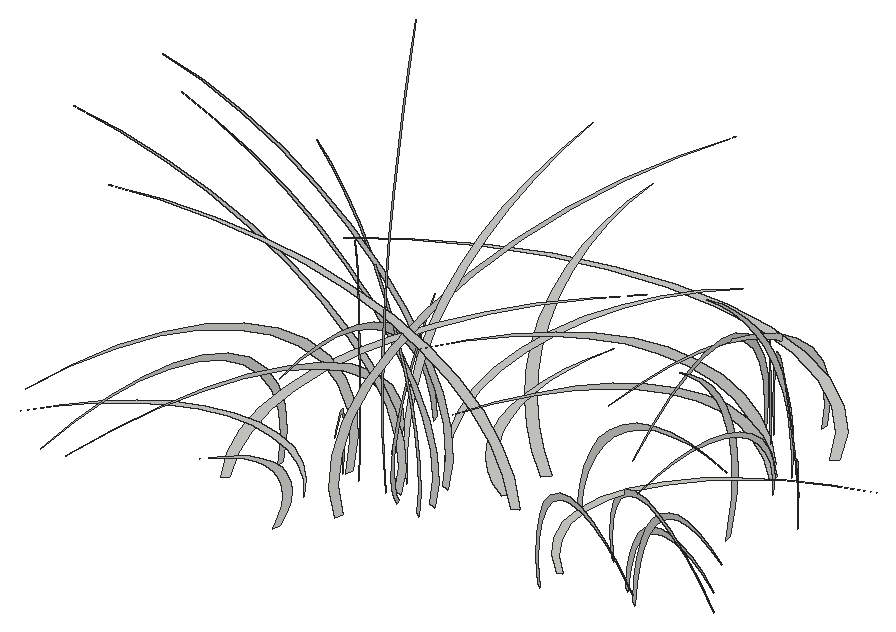
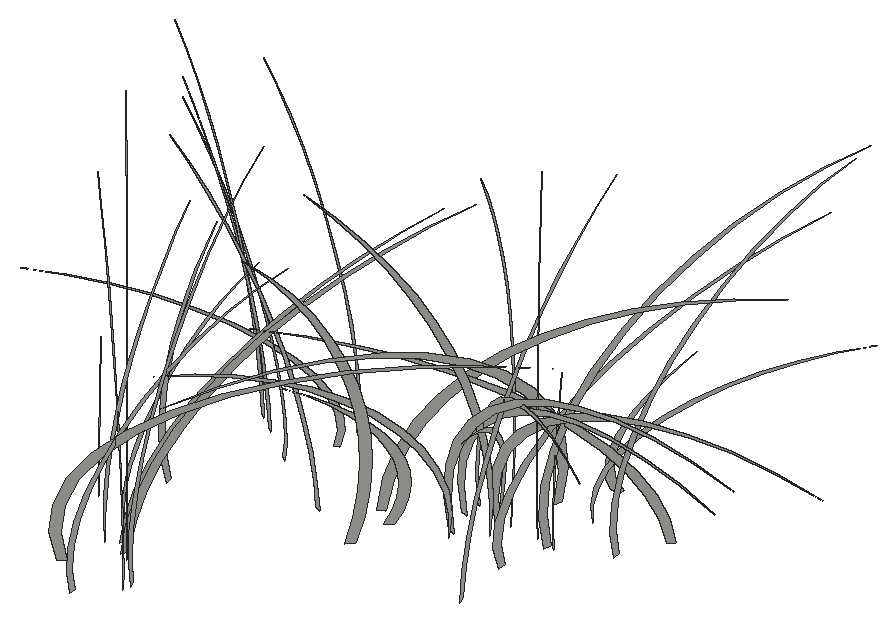
# SketchUp Ruby script. Lengths in inches.
U = 1.inch
M = Sketchup.active_model
def pt(a) = Geom::Point3d.new(a.map { |v| v * U })
def face(e, loops, mat)
  f = e.add_face(loops[0].map { |a| pt(a) })
  loops[1..].each { |l| e.add_face(l.map { |a| pt(a) }).erase! }
  f.material = f.back_material = mat if mat
  f
end
# faces: each face lists its corners as indices into pts; further lists are holes
def faces(e, pts, list, mat = nil) = list.each { |f| face(e, (f[0].is_a?(Array) ? f : [f]).map { |l| l.map { |i| pts[i] } }, mat) }
# xy, xz, yz: faces in a plane at the given z, y or x. An outline is a flat list of corners, or four numbers for a rectangle; further outlines are holes
def ring(l) = l.size == 4 ? [[l[0], l[1]], [l[2], l[1]], [l[2], l[3]], [l[0], l[3]]] : l.each_slice(2).to_a
def flat(e, list, mat, &to3) = list.each { |f| face(e, (f[0].is_a?(Array) ? f : [f]).map { |l| ring(l).map { |u, v| to3.(u, v) } }, mat) }
def xy(e, z, list, mat = nil) = flat(e, list, mat) { |x, y| [x, y, z] }
def xz(e, y, list, mat = nil) = flat(e, list, mat) { |x, z| [x, y, z] }
def yz(e, x, list, mat = nil) = flat(e, list, mat) { |y, z| [x, y, z] }
def lines(e, pts, list) = list.each { |a, b| e.add_line(pt(pts[a]), pt(pts[b])) }
# prism: a flat outline (further loops are holes) pulled along v
def prism(e, loops, v, mat = nil)
  f = face(e, loops, mat); d = Geom::Vector3d.new(v.map { |x| x * U })
  f.pushpull(f.normal.samedirection?(d) ? d.length : -d.length)
end
def box(e, o, s, mat = nil) = prism(e, [[o, [o[0] + s[0], o[1], o[2]], [o[0] + s[0], o[1] + s[1], o[2]], [o[0], o[1] + s[1], o[2]]]], [0, 0, s[2]], mat)
def at(x, y, z, deg = 0) = Geom::Transformation.translation(pt([x, y, z])) * Geom::Transformation.rotation(ORIGIN, Z_AXIS, deg.degrees)
def axes(o, x, y, z) = Geom::Transformation.new([*x, 0, *y, 0, *z, 0, *pt(o).to_a, 1])
def part(name) = M.definitions.add(name)
# library, detail: a bought-in or finely detailed component or shape, given as its bounding box
def library(name, o, s) = part(name).tap { |d| box(d.entities, o, s) }
def detail(e, o, s) = box(e.add_group.entities, o, s)
def put(e, d, t, mat = nil) = e.add_instance(d, t).tap { |i| i.material = mat if mat }
def group(e, t, mat = nil) = e.add_group.tap { |g| g.transformation = t; g.material = mat if mat }.entities
root = M.entities
g1 = group(root,at(58.66,562.84,0.02))
p = [[0.12,-0.92,0],[0.05,-0.41,0],[0,0,1.75],[0.02,-0.16,3.51],[0.11,-0.9,5.24],[0.27,-2.18,6.89],
  [0.5,-3.98,8.42],[0.79,-6.26,9.8],[1.13,-8.95,10.98],[1.51,-12,11.95],[1.93,-15.32,12.67],[2.37,-18.83,13.13],
  [2.83,-22.45,13.32],[3.28,-26.08,13.23],[2.84,-22.52,13.25],[2.39,-18.99,13],[1.96,-15.57,12.5],[1.56,-12.36,11.75],
  [1.19,-9.41,10.78],[0.86,-6.8,9.6],[0.58,-4.59,8.25],[0.36,-2.83,6.75],[0.2,-1.56,5.13],[0.1,-0.81,3.44],
  [0.07,-0.59,1.72]]
faces(g1,p,[[0,1,2,3,4,5,6,7,8,9,10,11,12,13,14,15,16,17,18,19,20,21,22,23,24]])
g2 = group(root,at(62.45,564.45,0.02))
p = [[-0.1,-0.92,0],[-0.05,-0.41,0],[0,0,2.0625],[-0.02,-0.17,4.13],[-0.1,-0.9,6.16],[-0.24,-2.1875,8.1],
  [-0.44,-3.99,9.91],[-0.69,-6.27,11.52],[-0.99,-8.97,12.92],[-1.33,-12.02,14.05],[-1.69,-15.34,14.9],[-2.08,-18.86,15.45],
  [-2.48,-22.49,15.67],[-2.88,-26.13,15.5625],[-2.49,-22.56,15.58],[-2.1,-19.02,15.29],[-1.72,-15.6,14.71],[-1.37,-12.38,13.83],
  [-1.04,-9.43,12.68],[-0.75,-6.81,11.3],[-0.51,-4.6,9.7],[-0.3125,-2.84,7.9375],[-0.17,-1.5625,6.04],[-0.09,-0.81,4.05],
  [-0.07,-0.59,2.02]]
faces(g2,p,[[0,1,2,3,4,5,6,7,8,9,10,11,12,13,14,15,16,17,18,19,20,21,22,23,24]])
g3 = group(root,at(62.45,564.45,0.02))
p = [[-0.1,-0.92,0],[-0.05,-0.41,0],[0,0,2.0625],[-0.02,-0.17,4.13],[-0.1,-0.9,6.16],[-0.24,-2.1875,8.1],
  [-0.44,-3.99,9.91],[-0.69,-6.27,11.52],[-0.99,-8.97,12.92],[-1.33,-12.02,14.05],[-1.69,-15.34,14.9],[-2.08,-18.86,15.45],
  [-2.48,-22.49,15.67],[-2.88,-26.13,15.5625],[-2.49,-22.56,15.58],[-2.1,-19.02,15.29],[-1.72,-15.6,14.71],[-1.37,-12.38,13.83],
  [-1.04,-9.43,12.68],[-0.75,-6.81,11.3],[-0.51,-4.6,9.7],[-0.3125,-2.84,7.9375],[-0.17,-1.5625,6.04],[-0.09,-0.81,4.05],
  [-0.07,-0.59,2.02]]
faces(g3,p,[[0,1,2,3,4,5,6,7,8,9,10,11,12,13,14,15,16,17,18,19,20,21,22,23,24]])
g4 = group(root,at(62.21,560.12,0.02))
p = [[-9.23,-14.04,8.41],[-7.99,-12.15,8.36],[-6.77,-10.29,8.15],[-5.59,-8.5,7.8],[-4.48,-6.8125,7.32],[-3.46,-5.26,6.7],
  [-2.54,-3.86,5.97],[-1.75,-2.66,5.13],[-1.09,-1.67,4.2],[-0.59,-0.9,3.21],[-0.25,-0.39,2.16],[-0.08,-0.125,1.09],
  [-0.08,-0.125,0],[0,0,1.11],[-0.11,-0.16,2.21],[-0.4,-0.61,3.29],[-0.88,-1.34,4.32],[-1.53,-2.33,5.28],
  [-2.33,-3.55,6.14],[-3.27,-4.98,6.88],[-4.33,-6.59,7.5],[-5.48,-8.34,7.97],[-6.7,-10.19,8.28],[-7.96,-12.11,8.43]]
faces(g4,p,[[0,1,2,3,4,5,6,7,8,9,10,11,12,13,14,15,16,17,18,19,20,21,22,23]])
g5 = group(root,at(78.25,560.67,0.02))
p = [[0.65,-0.5,0],[0.29,-0.22,0],[0,0,1.55],[0.12,-0.09,3.11],[0.63,-0.49,4.64],[1.54,-1.19,6.1],
  [2.81,-2.18,7.45],[4.41,-3.42,8.67],[6.31,-4.9,9.72],[8.45,-6.5625,10.57],[10.79,-8.38,11.21],[13.27,-10.3,11.62],
  [15.82,-12.28,11.79],[18.375,-14.26,11.71],[15.86,-12.31,11.72],[13.375,-10.38,11.5],[10.97,-8.52,11.0625],[8.71,-6.76,10.4],
  [6.63,-5.15,9.54],[4.79,-3.72,8.5],[3.24,-2.51,7.3],[1.99,-1.55,5.97],[1.1,-0.85,4.54],[0.57,-0.44,3.05],
  [0.42,-0.32,1.52]]
faces(g5,p,[[0,1,2,3,4,5,6,7,8,9,10,11,12,13,14,15,16,17,18,19,20,21,22,23,24]])
g6 = group(root,at(63,567.87,0.02))
p = [[-0.06,-0.99,0],[-0.03,-0.44,0],[0,0,1.49],[-0.01,-0.18,2.99],[-0.06,-0.97,4.45],[-0.14,-2.36,5.86],
  [-0.26,-4.3,7.16],[-0.4,-6.76,8.33],[-0.58,-9.67,9.33],[-0.77,-12.96,10.15],[-0.99,-16.54,10.77],[-1.22,-20.34,11.16],
  [-1.45,-24.24,11.32],[-1.68,-28.17,11.24],[-1.45,-24.32,11.26],[-1.23,-20.51,11.05],[-1.01,-16.82,10.625],[-0.8,-13.35,9.99],
  [-0.61,-10.16,9.16],[-0.4375,-7.35,8.16],[-0.3,-4.96,7.01],[-0.18,-3.06,5.73],[-0.1,-1.69,4.36],[-0.05,-0.87,2.93],
  [-0.04,-0.64,1.46]]
faces(g6,p,[[0,1,2,3,4,5,6,7,8,9,10,11,12,13,14,15,16,17,18,19,20,21,22,23,24]])
g7 = group(root,at(63.25,557.55,0.02))
p = [[-0.91,-7.12,6.7],[-0.75,-5.82,6.27],[-0.6,-4.64,5.81],[-0.46,-3.6,5.31],[-0.35,-2.71,4.77],[-0.25,-1.97,4.21],
  [-0.18,-1.39,3.63],[-0.125,-0.98,3.03],[-0.09,-0.74,2.43],[-0.09,-0.67,1.8125],[-0.1,-0.77,1.2],[-0.13,-1.05,0.59],
  [-0.19,-1.49,0],[-0.12,-0.92,0],[-0.05,-0.42,0.6],[-0.01,-0.11,1.22],[0,0,1.84],[-0.01,-0.08,2.47],
  [-0.04,-0.35,3.09],[-0.1,-0.81,3.69],[-0.1875,-1.45,4.28],[-0.29,-2.27,4.84],[-0.42,-3.26,5.37],[-0.57,-4.41,5.86],
  [-0.73,-5.7,6.3]]
faces(g7,p,[[0,1,2,3,4,5,6,7,8,9,10,11,12,13,14,15,16,17,18,19,20,21,22,23,24]])
g8 = group(root,at(84,562.16,0.02))
p = [[14.52,-11.27,13.58],[16.72,-12.98,13.9375],[14.59,-11.33,13.5],[12.54,-9.74,12.9],[10.59,-8.22,12.14],[8.75,-6.79,11.23],
  [7.05,-5.48,10.18],[5.51,-4.28,8.99],[4.14,-3.22,7.7],[2.97,-2.3,6.29],[1.99,-1.55,4.81],[1.23,-0.95,3.25],
  [0.69,-0.54,1.64],[0.38,-0.29,0],[0,0,0],[0.26,-0.2,1.68],[0.76,-0.59,3.33],[1.51,-1.17,4.92],
  [2.49,-1.93,6.45],[3.69,-2.87,7.875],[5.1,-3.96,9.19],[6.7,-5.2,10.38],[8.46,-6.57,11.43],[10.37,-8.05,12.3125],
  [12.4,-9.625,13.03]]
faces(g8,p,[[0,1,2,3,4,5,6,7,8,9,10,11,12,13,14,15,16,17,18,19,20,21,22,23,24]])
g9 = group(root,at(82.65,563.21,0.02))
p = [[14.52,-11.27,10.95],[16.72,-12.98,11.24],[14.59,-11.33,10.89],[12.54,-9.74,10.41],[10.59,-8.22,9.79],[8.75,-6.79,9.06],
  [7.05,-5.48,8.21],[5.51,-4.28,7.25],[4.14,-3.22,6.21],[2.97,-2.3,5.08],[1.99,-1.55,3.875],[1.23,-0.95,2.62],
  [0.69,-0.54,1.32],[0.38,-0.29,0],[0,0,0],[0.26,-0.2,1.36],[0.76,-0.59,2.69],[1.51,-1.17,3.97],
  [2.49,-1.93,5.2],[3.69,-2.87,6.35],[5.1,-3.96,7.41],[6.7,-5.2,8.37],[8.46,-6.57,9.21],[10.37,-8.05,9.93],
  [12.4,-9.625,10.51]]
faces(g9,p,[[0,1,2,3,4,5,6,7,8,9,10,11,12,13,14,15,16,17,18,19,20,21,22,23,24]])
g10 = group(root,at(79.64,565.54,0.02))
p = [[0.69,-0.54,0],[0.31,-0.24,0],[0,0,1.32],[0.125,-0.1,2.64],[0.68,-0.53,3.94],[1.65,-1.28,5.18],
  [3.01,-2.34,6.33],[4.74,-3.68,7.37],[6.77,-5.26,8.26],[9.07,-7.04,8.99],[11.59,-8.99,9.53],[14.24,-11.06,9.875],
  [16.98,-13.18,10.02],[19.73,-15.3125,9.95],[17.03,-13.22,9.96],[14.36,-11.15,9.78],[11.78,-9.14,9.4],[9.35,-7.26,8.84],
  [7.12,-5.53,8.11],[5.15,-3.99,7.22],[3.47,-2.7,6.2],[2.14,-1.66,5.07],[1.18,-0.92,3.86],[0.61,-0.47,2.59],
  [0.45,-0.35,1.29]]
faces(g10,p,[[0,1,2,3,4,5,6,7,8,9,10,11,12,13,14,15,16,17,18,19,20,21,22,23,24]])
g11 = group(root,at(62.26,571.81,0.02))
p = [[6.07,-19.87,14.56],[6.99,-22.87,14.94],[6.1,-19.96,14.48],[5.25,-17.16,13.83],[4.43,-14.49,13.02],[3.66,-11.97,12.04],
  [2.95,-9.65,10.91],[2.31,-7.54,9.64],[1.73,-5.67,8.25],[1.24,-4.06,6.75],[0.83,-2.72,5.15],[0.51,-1.68,3.49],
  [0.29,-0.94,1.76],[0.16,-0.52,0],[0,0,0],[0.11,-0.35,1.8],[0.32,-1.04,3.57],[0.63,-2.07,5.28],
  [1.04,-3.41,6.91],[1.55,-5.05,8.44],[2.13,-6.98,9.85],[2.8,-9.16,11.13],[3.54,-11.58,12.25],[4.34,-14.1875,13.2],
  [5.1875,-16.96,13.97]]
faces(g11,p,[[0,1,2,3,4,5,6,7,8,9,10,11,12,13,14,15,16,17,18,19,20,21,22,23,24]])
g12 = group(root,at(62.8125,564.18,0.02))
p = [[0.57,-0.76,0],[0.25,-0.34,1.67],[0.0625,-0.09,3.36],[0,0,5.0625],[0.0625,-0.08,6.76],[0.25,-0.33,8.45],
  [0.5625,-0.75,10.12],[1,-1.34,11.77],[1.56,-2.08,13.4],[2.23,-2.99,14.98],[3.03,-4.05,16.53],[3.93,-5.26,18.02],
  [4.95,-6.62,19.46],[3.99,-5.34,18],[3.14,-4.2,16.49],[2.39,-3.19,14.9375],[1.74,-2.33,13.35],[1.2,-1.61,11.73],
  [0.77,-1.03,10.08],[0.46,-0.61,8.42],[0.25,-0.34,6.74],[0.16,-0.21,5.05],[0.18,-0.24,3.36],[0.32,-0.43,1.68]]
faces(g12,p,[[0,1,2,3,4,5,6,7,8,9,10,11,12,13,14,15,16,17,18,19,20,21,22,23]])
g13 = group(root,at(61.19,564.82,0.02))
p = [[5.52,-7.72,6.7],[4.47,-6.25,6.27],[3.52,-4.92,5.81],[2.68,-3.75,5.31],[1.96,-2.74,4.77],[1.37,-1.91,4.21],
  [0.9,-1.26,3.63],[0.57,-0.79,3.03],[0.37,-0.52,2.43],[0.31,-0.44,1.8125],[0.4,-0.56,1.2],[0.62,-0.87,0.59],
  [0.98,-1.37,0],[0.74,-1.03,0],[0.33,-0.46,0.59],[0.07,-0.1,1.19],[-0.04,0.05,1.81],[0.01,-0.02,2.43],
  [0.21,-0.3,3.04],[0.5625,-0.79,3.65],[1.0625,-1.49,4.23],[1.7,-2.38,4.8],[2.48,-3.47,5.33],[3.38,-4.73,5.83],
  [4.4,-6.15,6.29]]
faces(g13,p,[[0,1,2,3,4,5,6,7,8,9,10,11,12,13,14,15,16,17,18,19,20,21,22,23,24]])
g14 = group(root,at(72.51,566.4,0.02))
p = [[-19.18,-7.98,16.73],[-22.08,-9.1875,17.17],[-19.27,-8.02,16.64],[-16.57,-6.9,15.9],[-13.98,-5.82,14.96],[-11.56,-4.8125,13.84],
  [-9.32,-3.88,12.54],[-7.28,-3.03,11.08],[-5.47,-2.28,9.48],[-3.92,-1.63,7.76],[-2.63,-1.09,5.92],[-1.625,-0.68,4.01],
  [-0.91,-0.38,2.02],[-0.5,-0.21,0],[0,0,0],[-0.34,-0.14,2.07],[-1.01,-0.42,4.1],[-1.99,-0.83,6.07],
  [-3.29,-1.37,7.94],[-4.88,-2.03,9.7],[-6.74,-2.81,11.33],[-8.85,-3.68,12.79],[-11.18,-4.65,14.08],[-13.7,-5.7,15.17],
  [-16.375,-6.82,16.0625]]
faces(g14,p,[[0,1,2,3,4,5,6,7,8,9,10,11,12,13,14,15,16,17,18,19,20,21,22,23,24]])
g15 = group(root,at(74.89,568.54,0.02))
p = [[16.23,-8.63,12.88],[18.68,-9.93,13.22],[16.3125,-8.67,12.8125],[14.02,-7.45,12.24],[11.84,-6.29,11.52],[9.78,-5.2,10.66],
  [7.88,-4.19,9.66],[6.16,-3.28,8.53],[4.63,-2.46,7.3],[3.32,-1.76,5.97],[2.23,-1.18,4.5625],[1.375,-0.73,3.08],
  [0.77,-0.41,1.56],[0.42,-0.22,0],[0,0,0],[0.29,-0.15,1.6],[0.85,-0.45,3.16],[1.6875,-0.9,4.67],
  [2.78,-1.48,6.12],[4.13,-2.2,7.47],[5.7,-3.03,8.72],[7.49,-3.98,9.85],[9.46,-5.03,10.84],[11.59,-6.16,11.68],
  [13.86,-7.37,12.37]]
faces(g15,p,[[0,1,2,3,4,5,6,7,8,9,10,11,12,13,14,15,16,17,18,19,20,21,22,23,24]])
g16 = group(root,at(78.28,562.01,0.02))
p = [[0.625,0.24,0],[0.28,0.11,0],[0,0,1.1],[0.11,0.04,2.21],[0.61,0.24,3.29],[1.49,0.57,4.33],
  [2.72,1.04,5.29],[4.28,1.64,6.15],[6.11,2.34,6.9],[8.19,3.14,7.51],[10.46,4.01,7.96],[12.86,4.93,8.25],
  [15.33,5.88,8.37],[17.8125,6.83,8.3125],[15.375,5.9,8.32],[12.97,4.97,8.17],[10.64,4.08,7.85],[8.4375,3.24,7.39],
  [6.43,2.46,6.77],[4.65,1.78,6.03],[3.14,1.2,5.18],[1.93,0.74,4.24],[1.07,0.41,3.23],[0.55,0.21,2.16],
  [0.4,0.16,1.08]]
faces(g16,p,[[0,1,2,3,4,5,6,7,8,9,10,11,12,13,14,15,16,17,18,19,20,21,22,23,24]])
g17 = group(root,at(57.05,558.92,0.02))
p = [[17.17,11.7,12.375],[19.76,13.47,12.7],[17.25,11.76,12.31],[14.83,10.11,11.76],[12.52,8.53,11.07],[10.35,7.05,10.23],
  [8.34,5.68,9.27],[6.52,4.44,8.2],[4.9,3.34,7.01],[3.51,2.39,5.74],[2.35,1.6,4.38],[1.45,0.99,2.96],
  [0.82,0.56,1.5],[0.45,0.3,0],[0,0,0],[0.3,0.21,1.53],[0.9,0.61,3.03],[1.78,1.22,4.49],
  [2.95,2.01,5.875],[4.37,2.98,7.18],[6.03,4.11,8.375],[7.92,5.4,9.46],[10,6.82,10.41],[12.26,8.36,11.22],
  [14.66,9.99,11.88]]
faces(g17,p,[[0,1,2,3,4,5,6,7,8,9,10,11,12,13,14,15,16,17,18,19,20,21,22,23,24]])
g18 = group(root,at(67.26,561.45,0.02))
p = [[-3.85,8.68,9.0625],[-3.11,7.03,8.49],[-2.45,5.54,7.85],[-1.87,4.22,7.18],[-1.37,3.08,6.45],[-0.95,2.15,5.7],
  [-0.625,1.41,4.91],[-0.39,0.89,4.1],[-0.26,0.58,3.28],[-0.22,0.49,2.45],[-0.28,0.625,1.625],[-0.43,0.97,0.8],
  [-0.68,1.54,0],[-0.52,1.16,0],[-0.23,0.52,0.8],[-0.05,0.11,1.61],[0.02,-0.06,2.45],[-0.01,0.02,3.28],
  [-0.15,0.33,4.11],[-0.39,0.89,4.93],[-0.74,1.67,5.72],[-1.1875,2.68,6.49],[-1.73,3.9,7.21],[-2.35,5.3125,7.88],
  [-3.0625,6.91,8.5]]
faces(g18,p,[[0,1,2,3,4,5,6,7,8,9,10,11,12,13,14,15,16,17,18,19,20,21,22,23,24]])
g19 = group(root,at(66.6875,563.51,0.02))
p = [[-0.98,0.17,0],[-0.43,0.08,0],[0,0,1.75],[-0.18,0.03,3.51],[-0.96,0.17,5.24],[-2.32,0.41,6.89],
  [-4.24,0.76,8.42],[-6.67,1.1875,9.8],[-9.54,1.7,10.98],[-12.78,2.28,11.95],[-16.32,2.91,12.67],[-20.06,3.57,13.13],
  [-23.91,4.26,13.32],[-27.78,4.95,13.23],[-23.98,4.27,13.25],[-20.22,3.6,13],[-16.59,2.96,12.5],[-13.16,2.34,11.75],
  [-10.02,1.79,10.78],[-7.25,1.29,9.6],[-4.89,0.87,8.25],[-3.02,0.54,6.75],[-1.66,0.3,5.13],[-0.86,0.15,3.44],
  [-0.63,0.11,1.72]]
faces(g19,p,[[0,1,2,3,4,5,6,7,8,9,10,11,12,13,14,15,16,17,18,19,20,21,22,23,24]])
g20 = group(root,at(66.6875,563.51,0.02))
p = [[-0.98,0.17,0],[-0.43,0.08,0],[0,0,1.75],[-0.18,0.03,3.51],[-0.96,0.17,5.24],[-2.32,0.41,6.89],
  [-4.24,0.76,8.42],[-6.67,1.1875,9.8],[-9.54,1.7,10.98],[-12.78,2.28,11.95],[-16.32,2.91,12.67],[-20.06,3.57,13.13],
  [-23.91,4.26,13.32],[-27.78,4.95,13.23],[-23.98,4.27,13.25],[-20.22,3.6,13],[-16.59,2.96,12.5],[-13.16,2.34,11.75],
  [-10.02,1.79,10.78],[-7.25,1.29,9.6],[-4.89,0.87,8.25],[-3.02,0.54,6.75],[-1.66,0.3,5.13],[-0.86,0.15,3.44],
  [-0.63,0.11,1.72]]
faces(g20,p,[[0,1,2,3,4,5,6,7,8,9,10,11,12,13,14,15,16,17,18,19,20,21,22,23,24]])
g21 = group(root,at(65.8,562.41,0.02))
p = [[-0.4,0.86,0],[-0.18,0.38,2.26],[-0.05,0.1,4.55],[0,0,6.84],[-0.04,0.09,9.14],[-0.18,0.38,11.42],
  [-0.4,0.85,13.6875],[-0.71,1.51,15.92],[-1.1,2.36,18.12],[-1.58,3.38,20.26],[-2.14,4.58,22.35],[-2.79,5.95,24.37],
  [-3.51,7.48,26.3125],[-2.83,6.04,24.34],[-2.22,4.75,22.3],[-1.69,3.61,20.2],[-1.23,2.63,18.05],[-0.85,1.82,15.86],
  [-0.55,1.17,13.64],[-0.32,0.6875,11.38],[-0.18,0.38,9.11],[-0.11,0.24,6.83],[-0.13,0.28,4.54],[-0.23,0.48,2.27]]
faces(g21,p,[[0,1,2,3,4,5,6,7,8,9,10,11,12,13,14,15,16,17,18,19,20,21,22,23]])
g22 = group(root,at(81.36,578.37,0.02))
p = [[-3.87,-20.41,12.375],[-4.45,-23.49,12.7],[-3.88,-20.51,12.31],[-3.34,-17.63,11.76],[-2.82,-14.88,11.07],[-2.33,-12.3,10.23],
  [-1.88,-9.91,9.27],[-1.47,-7.75,8.2],[-1.1,-5.82,7.01],[-0.79,-4.17,5.74],[-0.53,-2.8,4.38],[-0.33,-1.73,2.96],
  [-0.18,-0.97,1.5],[-0.1,-0.53,0],[0,0,0],[-0.07,-0.36,1.53],[-0.2,-1.07,3.03],[-0.4,-2.12,4.49],
  [-0.66,-3.5,5.875],[-0.98,-5.19,7.18],[-1.36,-7.17,8.375],[-1.78,-9.42,9.46],[-2.25,-11.89,10.41],[-2.76,-14.58,11.22],
  [-3.3,-17.43,11.88]]
faces(g22,p,[[0,1,2,3,4,5,6,7,8,9,10,11,12,13,14,15,16,17,18,19,20,21,22,23,24]])
g23 = group(root,at(80.5,579.34,0.02))
p = [[-6.28,-19.8,14.56],[-7.23,-22.79,14.94],[-6.3125,-19.9,14.48],[-5.43,-17.1,13.83],[-4.58,-14.4375,13.02],[-3.79,-11.93,12.04],
  [-3.05,-9.62,10.91],[-2.38,-7.52,9.64],[-1.79,-5.65,8.25],[-1.28,-4.04,6.75],[-0.86,-2.71,5.15],[-0.53,-1.68,3.49],
  [-0.3,-0.94,1.76],[-0.16,-0.52,0],[0,0,0],[-0.11,-0.35,1.8],[-0.33,-1.04,3.57],[-0.65,-2.06,5.28],
  [-1.08,-3.4,6.91],[-1.6,-5.04,8.44],[-2.21,-6.96,9.85],[-2.9,-9.13,11.13],[-3.66,-11.54,12.25],[-4.49,-14.14,13.2],
  [-5.36,-16.91,13.97]]
faces(g23,p,[[0,1,2,3,4,5,6,7,8,9,10,11,12,13,14,15,16,17,18,19,20,21,22,23,24]])
g24 = group(root,at(80.5,579.34,0.02))
p = [[-6.28,-19.8,14.56],[-7.23,-22.79,14.94],[-6.3125,-19.9,14.48],[-5.43,-17.1,13.83],[-4.58,-14.4375,13.02],[-3.79,-11.93,12.04],
  [-3.05,-9.62,10.91],[-2.38,-7.52,9.64],[-1.79,-5.65,8.25],[-1.28,-4.04,6.75],[-0.86,-2.71,5.15],[-0.53,-1.68,3.49],
  [-0.3,-0.94,1.76],[-0.16,-0.52,0],[0,0,0],[-0.11,-0.35,1.8],[-0.33,-1.04,3.57],[-0.65,-2.06,5.28],
  [-1.08,-3.4,6.91],[-1.6,-5.04,8.44],[-2.21,-6.96,9.85],[-2.9,-9.13,11.13],[-3.66,-11.54,12.25],[-4.49,-14.14,13.2],
  [-5.36,-16.91,13.97]]
faces(g24,p,[[0,1,2,3,4,5,6,7,8,9,10,11,12,13,14,15,16,17,18,19,20,21,22,23,24]])
g25 = group(root,at(68.87,562.08,0.02))
p = [[-0.62,0.44,0],[-0.27,0.2,0],[0,0,1.68],[-0.11,0.08,3.37],[-0.6,0.43,5.03],[-1.46,1.05,6.61],
  [-2.67,1.92,8.08],[-4.2,3.02,9.4],[-6.01,4.32,10.54],[-8.05,5.79,11.47],[-10.28,7.39,12.16],[-12.64,9.08,12.61],
  [-15.07,10.83,12.79],[-17.5,12.58,12.7],[-15.11,10.86,12.72],[-12.74,9.16,12.48],[-10.45,7.51,12],[-8.29,5.96,11.29],
  [-6.32,4.54,10.35],[-4.57,3.28,9.22],[-3.08,2.21,7.92],[-1.9,1.37,6.48],[-1.05,0.75,4.93],[-0.54,0.39,3.31],
  [-0.4,0.29,1.65]]
faces(g25,p,[[0,1,2,3,4,5,6,7,8,9,10,11,12,13,14,15,16,17,18,19,20,21,22,23,24]])
g26 = group(root,at(65.61,564.66,0.02))
p = [[7.51,7.51,22.54],[6.3125,6.3125,20.88],[5.21,5.21,19.16],[4.21,4.21,17.39],[3.32,3.32,15.57],[2.52,2.52,13.71],
  [1.84,1.84,11.82],[1.27,1.27,9.89],[0.81,0.81,7.94],[0.46,0.46,5.97],[0.22,0.22,3.99],[0.1,0.1,2],
  [0.1,0.1,0],[0,0,2.01],[0.04,0.04,4.01],[0.21,0.21,6.01],[0.51,0.51,8],[0.95,0.95,9.97],
  [1.51,1.51,11.91],[2.21,2.21,13.81],[3.03,3.03,15.67],[3.98,3.98,17.48],[5.04,5.04,19.23],[6.22,6.22,20.92]]
faces(g26,p,[[0,1,2,3,4,5,6,7,8,9,10,11,12,13,14,15,16,17,18,19,20,21,22,23]])
g27 = group(root,at(69.03,563.47,0.02))
p = [[-0.93,0.35,0],[-0.41,0.16,0],[0,0,1.75],[-0.17,0.0625,3.51],[-0.91,0.34,5.24],[-2.21,0.83,6.89],
  [-4.03,1.52,8.42],[-6.34,2.39,9.8],[-9.0625,3.42,10.98],[-12.14,4.59,11.95],[-15.5,5.86,12.67],[-19.06,7.2,13.13],
  [-22.72,8.58,13.32],[-26.4,9.97,13.23],[-22.79,8.61,13.25],[-19.22,7.26,13],[-15.76,5.96,12.5],[-12.51,4.73,11.75],
  [-9.53,3.6,10.78],[-6.89,2.6,9.6],[-4.65,1.76,8.25],[-2.87,1.08,6.75],[-1.58,0.6,5.13],[-0.82,0.31,3.44],
  [-0.6,0.23,1.72]]
faces(g27,p,[[0,1,2,3,4,5,6,7,8,9,10,11,12,13,14,15,16,17,18,19,20,21,22,23,24]])
g28 = group(root,at(82.5,576.71,0.02))
p = [[3.4,-16.45,8.41],[2.94,-14.24,8.36],[2.49,-12.0625,8.15],[2.06,-9.96,7.8],[1.65,-7.98,7.32],[1.27,-6.16,6.7],
  [0.9375,-4.53,5.97],[0.64,-3.12,5.13],[0.4,-1.95,4.2],[0.22,-1.06,3.21],[0.09,-0.45,2.16],[0.03,-0.15,1.09],
  [0.03,-0.15,0],[0,0,1.11],[0.04,-0.19,2.21],[0.15,-0.72,3.29],[0.32,-1.57,4.32],[0.5625,-2.73,5.28],
  [0.86,-4.16,6.14],[1.21,-5.84,6.88],[1.6,-7.72,7.5],[2.02,-9.77,7.97],[2.47,-11.94,8.28],[2.93,-14.1875,8.43]]
faces(g28,p,[[0,1,2,3,4,5,6,7,8,9,10,11,12,13,14,15,16,17,18,19,20,21,22,23]])
g29 = group(root,at(83.41,572.28,0.02))
p = [[1.45,-7.03,13.62],[1.1875,-5.75,12.76],[0.95,-4.58,11.81],[0.74,-3.56,10.79],[0.55,-2.68,9.7],[0.4,-1.95,8.57],
  [0.28,-1.375,7.38],[0.2,-0.97,6.17],[0.15,-0.73,4.93],[0.14,-0.66,3.6875],[0.16,-0.76,2.44],[0.21,-1.03,1.21],
  [0.3,-1.47,0],[0.1875,-0.91,0],[0.09,-0.42,1.22],[0.02,-0.11,2.48],[0,0,3.75],[0.02,-0.08,5.02],
  [0.07,-0.34,6.28],[0.16,-0.8,7.51],[0.3,-1.43,8.7],[0.46,-2.24,9.84],[0.67,-3.22,10.91],[0.9,-4.35,11.9],
  [1.16,-5.625,12.8125]]
faces(g29,p,[[0,1,2,3,4,5,6,7,8,9,10,11,12,13,14,15,16,17,18,19,20,21,22,23,24]])
g30 = group(root,at(70.07,566.39,0.02))
p = [[5.08,5.08,9.0625],[4.15,4.15,8.49],[3.31,3.31,7.85],[2.57,2.57,7.18],[1.93,1.93,6.45],[1.41,1.41,5.7],
  [0.99,0.99,4.91],[0.7,0.7,4.1],[0.53,0.53,3.28],[0.48,0.48,2.45],[0.55,0.55,1.625],[0.75,0.75,0.8],
  [1.0625,1.0625,0],[0.65,0.65,0],[0.3,0.3,0.81],[0.08,0.08,1.65],[0,0,2.49],[0.06,0.06,3.34],
  [0.25,0.25,4.17],[0.58,0.58,4.99],[1.04,1.04,5.79],[1.62,1.62,6.54],[2.33,2.33,7.26],[3.14,3.14,7.92],
  [4.0625,4.0625,8.52]]
faces(g30,p,[[0,1,2,3,4,5,6,7,8,9,10,11,12,13,14,15,16,17,18,19,20,21,22,23,24]])
g31 = group(root,at(77.54,582.35,0.02))
p = [[0.39,-0.91,0],[0.17,-0.41,0],[0,0,1.75],[0.07,-0.16,3.51],[0.38,-0.89,5.24],[0.93,-2.17,6.89],
  [1.69,-3.97,8.42],[2.66,-6.23,9.8],[3.8,-8.91,10.98],[5.09,-11.94,11.95],[6.5,-15.24,12.67],[7.99,-18.74,13.13],
  [9.53,-22.34,13.32],[11.07,-25.96,13.23],[9.56,-22.41,13.25],[8.06,-18.9,13],[6.61,-15.5,12.5],[5.25,-12.3,11.75],
  [3.99,-9.37,10.78],[2.89,-6.77,9.6],[1.95,-4.57,8.25],[1.2,-2.82,6.75],[0.66,-1.55,5.13],[0.34,-0.8,3.44],
  [0.25,-0.59,1.72]]
faces(g31,p,[[0,1,2,3,4,5,6,7,8,9,10,11,12,13,14,15,16,17,18,19,20,21,22,23,24]])
g32 = group(root,at(68.37,565.55,0.02))
p = [[-0.95,0.28,0],[-0.42,0.125,0],[0,0,2.01],[-0.17,0.05,4.04],[-0.93,0.27,6.02],[-2.27,0.66,7.92],
  [-4.14,1.21,9.68],[-6.5,1.9,11.26],[-9.3,2.72,12.62],[-12.46,3.64,13.73],[-15.91,4.65,14.5625],[-19.55,5.72,15.09],
  [-23.3125,6.82,15.31],[-27.08,7.92,15.2],[-23.38,6.84,15.22],[-19.72,5.77,14.94],[-16.17,4.73,14.37],[-12.83,3.75,13.51],
  [-9.77,2.86,12.39],[-7.0625,2.07,11.04],[-4.77,1.39,9.48],[-2.94,0.86,7.75],[-1.62,0.47,5.9],[-0.84,0.25,3.96],
  [-0.61,0.18,1.98]]
faces(g32,p,[[0,1,2,3,4,5,6,7,8,9,10,11,12,13,14,15,16,17,18,19,20,21,22,23,24]])
g33 = group(root,at(79.6,579.94,0.02))
p = [[0.58,-0.72,0],[0.26,-0.32,0],[0,0,2.0625],[0.1,-0.13,4.13],[0.57,-0.71,6.16],[1.375,-1.72,8.1],
  [2.51,-3.13,9.91],[3.95,-4.92,11.52],[5.64,-7.04,12.92],[7.5625,-9.4375,14.05],[9.65,-12.05,14.9],[11.87,-14.8125,15.45],
  [14.15,-17.66,15.67],[16.44,-20.51,15.5625],[14.1875,-17.71,15.58],[11.96,-14.93,15.29],[9.8125,-12.25,14.71],[7.79,-9.72,13.83],
  [5.93,-7.4,12.68],[4.29,-5.35,11.3],[2.89,-3.61,9.7],[1.78,-2.23,7.9375],[0.98,-1.23,6.04],[0.51,-0.64,4.05],
  [0.375,-0.47,2.02]]
faces(g33,p,[[0,1,2,3,4,5,6,7,8,9,10,11,12,13,14,15,16,17,18,19,20,21,22,23,24]])
g34 = group(root,at(79.6,579.94,0.02))
p = [[0.58,-0.72,0],[0.26,-0.32,0],[0,0,2.0625],[0.1,-0.13,4.13],[0.57,-0.71,6.16],[1.375,-1.72,8.1],
  [2.51,-3.13,9.91],[3.95,-4.92,11.52],[5.64,-7.04,12.92],[7.5625,-9.4375,14.05],[9.65,-12.05,14.9],[11.87,-14.8125,15.45],
  [14.15,-17.66,15.67],[16.44,-20.51,15.5625],[14.1875,-17.71,15.58],[11.96,-14.93,15.29],[9.8125,-12.25,14.71],[7.79,-9.72,13.83],
  [5.93,-7.4,12.68],[4.29,-5.35,11.3],[2.89,-3.61,9.7],[1.78,-2.23,7.9375],[0.98,-1.23,6.04],[0.51,-0.64,4.05],
  [0.375,-0.47,2.02]]
faces(g34,p,[[0,1,2,3,4,5,6,7,8,9,10,11,12,13,14,15,16,17,18,19,20,21,22,23,24]])
g35 = group(root,at(70.41,569.46,0.02))
p = [[5.08,5.08,18.42],[4.15,4.15,17.25],[3.31,3.31,15.97],[2.57,2.57,14.59],[1.93,1.93,13.12],[1.41,1.41,11.58],
  [0.99,0.99,9.98],[0.7,0.7,8.34],[0.53,0.53,6.67],[0.48,0.48,4.99],[0.55,0.55,3.3],[0.75,0.75,1.63],
  [1.0625,1.0625,0],[0.65,0.65,0],[0.3,0.3,1.66],[0.08,0.08,3.35],[0,0,5.07],[0.06,0.06,6.79],
  [0.25,0.25,8.49],[0.58,0.58,10.15],[1.04,1.04,11.76],[1.62,1.62,13.3],[2.33,2.33,14.75],[3.14,3.14,16.1],
  [4.0625,4.0625,17.33]]
faces(g35,p,[[0,1,2,3,4,5,6,7,8,9,10,11,12,13,14,15,16,17,18,19,20,21,22,23,24]])
g36 = group(root,at(77.58,582.75,0.02))
p = [[0.66,-0.74,0],[0.29,-0.33,0],[0,0,1.49],[0.12,-0.13,2.99],[0.65,-0.73,4.45],[1.57,-1.77,5.86],
  [2.86,-3.22,7.16],[4.5,-5.07,8.33],[6.43,-7.25,9.33],[8.62,-9.71,10.15],[11,-12.4,10.77],[13.52,-15.24,11.16],
  [16.12,-18.17,11.32],[18.73,-21.11,11.24],[16.17,-18.22,11.26],[13.63,-15.37,11.05],[11.18,-12.6,10.625],[8.875,-10,9.99],
  [6.76,-7.62,9.16],[4.88,-5.51,8.16],[3.3,-3.72,7.01],[2.03,-2.29,5.73],[1.12,-1.26,4.36],[0.58,-0.65,2.93],
  [0.43,-0.48,1.46]]
faces(g36,p,[[0,1,2,3,4,5,6,7,8,9,10,11,12,13,14,15,16,17,18,19,20,21,22,23,24]])
g37 = group(root,at(67.22,566.27,0.02))
p = [[11.88,11.88,11.375],[10.28,10.28,11.3],[8.71,8.71,11.03],[7.19,7.19,10.55],[5.77,5.77,9.89],[4.45,4.45,9.0625],
  [3.27,3.27,8.07],[2.25,2.25,6.9375],[1.41,1.41,5.69],[0.76,0.76,4.34],[0.33,0.33,2.93],[0.11,0.11,1.47],
  [0.11,0.11,0],[0,0,1.5],[0.14,0.14,3],[0.52,0.52,4.46],[1.13,1.13,5.85],[1.97,1.97,7.14],
  [3,3,8.3],[4.21,4.21,9.31],[5.58,5.58,10.14],[7.06,7.06,10.77],[8.625,8.625,11.19],[10.24,10.24,11.4]]
faces(g37,p,[[0,1,2,3,4,5,6,7,8,9,10,11,12,13,14,15,16,17,18,19,20,21,22,23]])
g38 = group(root,at(64.875,558.84,0.02))
p = [[0.26,0.96,0],[0.11,0.43,0],[0,0,2.01],[0.05,0.17,4.04],[0.25,0.9375,6.02],[0.62,2.28,7.92],
  [1.125,4.16,9.68],[1.76,6.54,11.26],[2.52,9.35,12.62],[3.38,12.53,13.73],[4.32,16,14.5625],[5.31,19.67,15.09],
  [6.33,23.45,15.31],[7.35,27.24,15.2],[6.35,23.52,15.22],[5.35,19.83,14.94],[4.39,16.27,14.37],[3.48,12.91,13.51],
  [2.65,9.83,12.39],[1.92,7.11,11.04],[1.29,4.8,9.48],[0.8,2.96,7.75],[0.44,1.63,5.9],[0.23,0.84,3.96],
  [0.17,0.62,1.98]]
faces(g38,p,[[0,1,2,3,4,5,6,7,8,9,10,11,12,13,14,15,16,17,18,19,20,21,22,23,24]])
g39 = group(root,at(85.05,575.625,0.02))
p = [[4.39,-5.68,6.7],[3.59,-4.64,6.27],[2.86,-3.7,5.81],[2.22,-2.875,5.31],[1.67,-2.16,4.77],[1.21,-1.57,4.21],
  [0.86,-1.11,3.63],[0.6,-0.78,3.03],[0.46,-0.59,2.43],[0.41,-0.53,1.8125],[0.48,-0.62,1.2],[0.64,-0.83,0.59],
  [0.92,-1.1875,0],[0.56,-0.73,0],[0.26,-0.34,0.6],[0.07,-0.09,1.22],[0,0,1.84],[0.05,-0.0625,2.47],
  [0.21,-0.28,3.09],[0.5,-0.64,3.69],[0.89,-1.16,4.28],[1.4,-1.8125,4.84],[2.01,-2.6,5.37],[2.72,-3.52,5.86],
  [3.51,-4.55,6.3]]
faces(g39,p,[[0,1,2,3,4,5,6,7,8,9,10,11,12,13,14,15,16,17,18,19,20,21,22,23,24]])
g40 = group(root,at(82.04,578.93,0.02))
p = [[2.15,-10.4,16.67],[1.81,-8.74,15.44],[1.49,-7.22,14.17],[1.21,-5.83,12.86],[0.95,-4.59,11.51],[0.72,-3.5,10.14],
  [0.53,-2.55,8.74],[0.36,-1.76,7.31],[0.23,-1.12,5.87],[0.13,-0.64,4.42],[0.0625,-0.31,2.95],[0.03,-0.14,1.48],
  [0.03,-0.14,0],[0,0,1.48],[0.01,-0.05,2.97],[0.06,-0.29,4.45],[0.15,-0.71,5.92],[0.27,-1.3125,7.37],
  [0.43,-2.1,8.81],[0.63,-3.0625,10.21],[0.87,-4.2,11.59],[1.14,-5.51,12.93],[1.44,-6.98,14.22],[1.78,-8.61,15.47]]
faces(g40,p,[[0,1,2,3,4,5,6,7,8,9,10,11,12,13,14,15,16,17,18,19,20,21,22,23]])
g41 = group(root,at(79.91,584.93,0.02))
p = [[0.05,-0.76,0],[0.02,-0.34,0],[0,0,1.46],[0.01,-0.14,2.93],[0.05,-0.74,4.375],[0.12,-1.8,5.75],
  [0.21,-3.29,7.03],[0.33,-5.16,8.18],[0.48,-7.38,9.17],[0.64,-9.9,9.98],[0.82,-12.63,10.58],[1,-15.53,10.97],
  [1.2,-18.51,11.125],[1.39,-21.51,11.05],[1.2,-18.57,11.0625],[1.01,-15.66,10.86],[0.83,-12.84,10.44],[0.66,-10.19,9.82],
  [0.5,-7.76,9.01],[0.36,-5.61,8.02],[0.24,-3.79,6.89],[0.15,-2.34,5.64],[0.08,-1.29,4.29],[0.04,-0.67,2.88],
  [0.03,-0.49,1.4375]]
faces(g41,p,[[0,1,2,3,4,5,6,7,8,9,10,11,12,13,14,15,16,17,18,19,20,21,22,23,24]])
g42 = group(root,at(83.27,582.28,0.02))
p = [[-0.8125,-0.57,0],[-0.36,-0.25,0],[0,0,1.75],[-0.15,-0.1,3.51],[-0.8,-0.56,5.24],[-1.9375,-1.35,6.89],
  [-3.54,-2.47,8.42],[-5.56,-3.875,9.8],[-7.95,-5.54,10.98],[-10.65,-7.43,11.95],[-13.59,-9.48,12.67],[-16.71,-11.66,13.13],
  [-19.92,-13.9,13.32],[-23.14,-16.15,13.23],[-19.98,-13.9375,13.25],[-16.85,-11.75,13],[-13.82,-9.64,12.5],[-10.97,-7.65,11.75],
  [-8.35,-5.83,10.78],[-6.04,-4.21,9.6],[-4.08,-2.84,8.25],[-2.51,-1.75,6.75],[-1.38,-0.97,5.13],[-0.72,-0.5,3.44],
  [-0.53,-0.37,1.72]]
faces(g42,p,[[0,1,2,3,4,5,6,7,8,9,10,11,12,13,14,15,16,17,18,19,20,21,22,23,24]])
g43 = group(root,at(83.27,582.28,0.02))
p = [[-0.8125,-0.57,0],[-0.36,-0.25,0],[0,0,1.75],[-0.15,-0.1,3.51],[-0.8,-0.56,5.24],[-1.9375,-1.35,6.89],
  [-3.54,-2.47,8.42],[-5.56,-3.875,9.8],[-7.95,-5.54,10.98],[-10.65,-7.43,11.95],[-13.59,-9.48,12.67],[-16.71,-11.66,13.13],
  [-19.92,-13.9,13.32],[-23.14,-16.15,13.23],[-19.98,-13.9375,13.25],[-16.85,-11.75,13],[-13.82,-9.64,12.5],[-10.97,-7.65,11.75],
  [-8.35,-5.83,10.78],[-6.04,-4.21,9.6],[-4.08,-2.84,8.25],[-2.51,-1.75,6.75],[-1.38,-0.97,5.13],[-0.72,-0.5,3.44],
  [-0.53,-0.37,1.72]]
faces(g43,p,[[0,1,2,3,4,5,6,7,8,9,10,11,12,13,14,15,16,17,18,19,20,21,22,23,24]])
